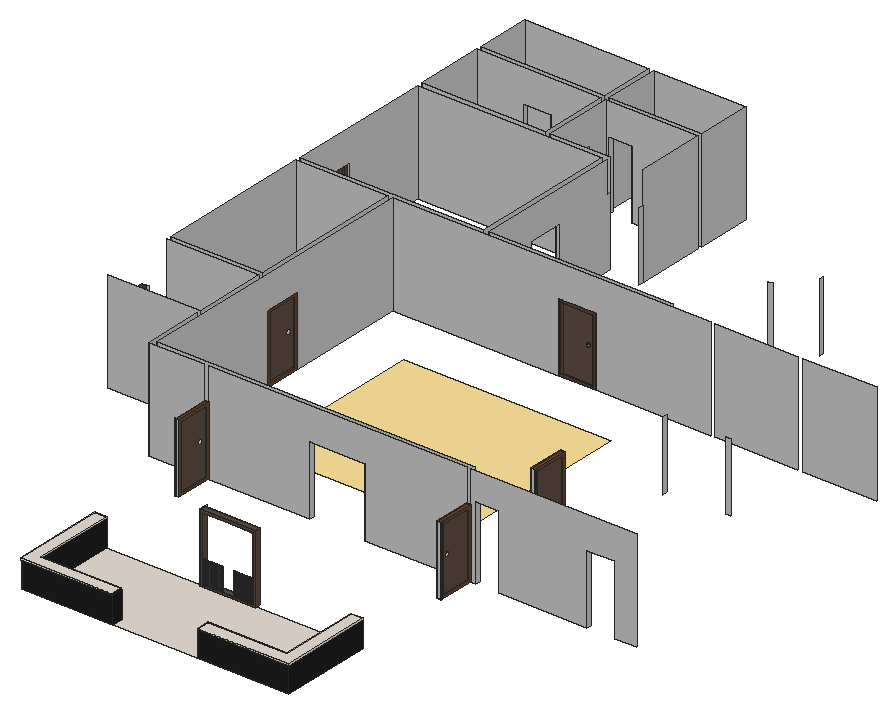
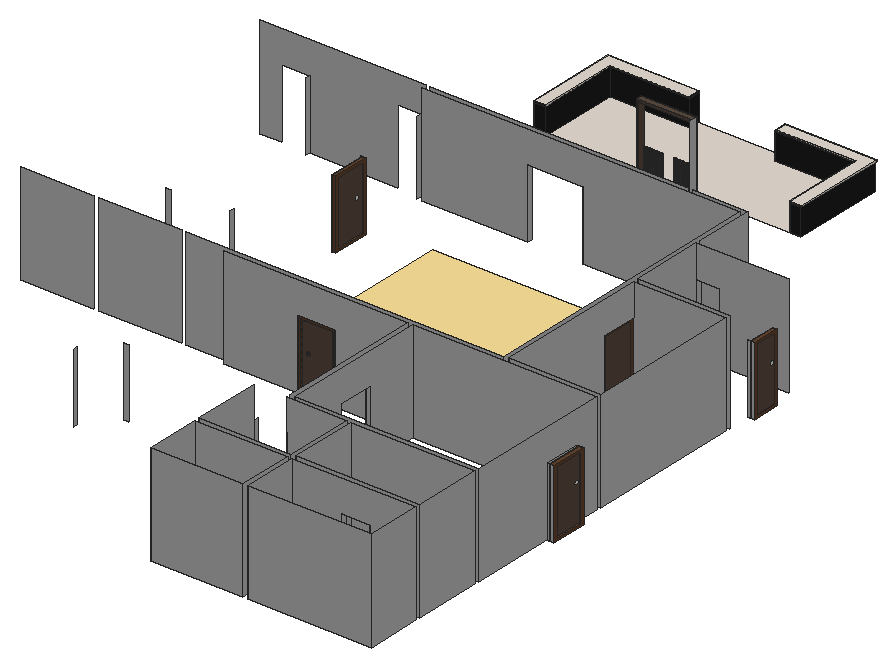
# SketchUp Ruby script. Lengths in inches.
U = 1.inch
M = Sketchup.active_model
def pt(a) = Geom::Point3d.new(a.map { |v| v * U })
def face(e, loops, mat)
  f = e.add_face(loops[0].map { |a| pt(a) })
  loops[1..].each { |l| e.add_face(l.map { |a| pt(a) }).erase! }
  f.material = f.back_material = mat if mat
  f
end
# faces: each face lists its corners as indices into pts; further lists are holes
def faces(e, pts, list, mat = nil) = list.each { |f| face(e, (f[0].is_a?(Array) ? f : [f]).map { |l| l.map { |i| pts[i] } }, mat) }
# xy, xz, yz: faces in a plane at the given z, y or x. An outline is a flat list of corners, or four numbers for a rectangle; further outlines are holes
def ring(l) = l.size == 4 ? [[l[0], l[1]], [l[2], l[1]], [l[2], l[3]], [l[0], l[3]]] : l.each_slice(2).to_a
def flat(e, list, mat, &to3) = list.each { |f| face(e, (f[0].is_a?(Array) ? f : [f]).map { |l| ring(l).map { |u, v| to3.(u, v) } }, mat) }
def xy(e, z, list, mat = nil) = flat(e, list, mat) { |x, y| [x, y, z] }
def xz(e, y, list, mat = nil) = flat(e, list, mat) { |x, z| [x, y, z] }
def yz(e, x, list, mat = nil) = flat(e, list, mat) { |y, z| [x, y, z] }
def lines(e, pts, list) = list.each { |a, b| e.add_line(pt(pts[a]), pt(pts[b])) }
# prism: a flat outline (further loops are holes) pulled along v
def prism(e, loops, v, mat = nil)
  f = face(e, loops, mat); d = Geom::Vector3d.new(v.map { |x| x * U })
  f.pushpull(f.normal.samedirection?(d) ? d.length : -d.length)
end
def box(e, o, s, mat = nil) = prism(e, [[o, [o[0] + s[0], o[1], o[2]], [o[0] + s[0], o[1] + s[1], o[2]], [o[0], o[1] + s[1], o[2]]]], [0, 0, s[2]], mat)
def at(x, y, z, deg = 0) = Geom::Transformation.translation(pt([x, y, z])) * Geom::Transformation.rotation(ORIGIN, Z_AXIS, deg.degrees)
def axes(o, x, y, z) = Geom::Transformation.new([*x, 0, *y, 0, *z, 0, *pt(o).to_a, 1])
def part(name) = M.definitions.add(name)
# library, detail: a bought-in or finely detailed component or shape, given as its bounding box
def library(name, o, s) = part(name).tap { |d| box(d.entities, o, s) }
def detail(e, o, s) = box(e.add_group.entities, o, s)
def put(e, d, t, mat = nil) = e.add_instance(d, t).tap { |i| i.material = mat if mat }
def group(e, t, mat = nil) = e.add_group.tap { |g| g.transformation = t; g.material = mat if mat }.entities
root = M.entities
M.materials.add("Brick_20_1K").color = [126, 109, 93]
M.materials.add("D02_Buttercup_Glow").color = [255, 229, 155]
M.materials.add("M02_Ash_Whisper").color = [196, 196, 196]
M.materials.add("M08_Obsidian_Black").color = [30, 30, 30]
M.materials.add("Marble_01_1K").color = [230, 221, 211]
M.materials.add("Metal_06_1K").color = [238, 236, 231]
M.materials.add("Wood_Floor_12_1K").color = [92, 75, 65]
M.materials.add("Wood_Planks_01_1K").color = [69, 67, 63]
M.materials.add("Wood_Veneer_15_1K").color = [103, 69, 45]
c1 = part("Group\#23")
box(c1.entities,[0,0,0],[0.6875,0.6875,26],"Wood_Planks_01_1K")
c2 = part("Group\#24")
box(c2.entities,[0,0,0],[0.6875,0.75,29.38],"Wood_Planks_01_1K")
c3 = part("Group\#19")
xy(c3.entities,0,[[0,-5,48,0]],"Wood_Veneer_15_1K")
xy(c3.entities,3,[[3,-5,45,-2],[3,-2,45,0]],"Wood_Veneer_15_1K")
xy(c3.entities,87,[[3,-5,45,-2],[3,-2,45,0]],"Wood_Veneer_15_1K")
xy(c3.entities,90,[[0,-5,48,0]],"Wood_Veneer_15_1K")
xz(c3.entities,-5,[[[0,0,48,90],[3,3,45,87]]],"Wood_Veneer_15_1K")
xz(c3.entities,-2,[[3,3,45,87]],"Wood_Floor_12_1K")
xz(c3.entities,0,[[[0,0,48,90],[3,3,45,87]]],"Wood_Veneer_15_1K")
yz(c3.entities,0,[[-5,0,0,90]],"Wood_Veneer_15_1K")
yz(c3.entities,3,[[-5,3,-2,87],[-2,3,0,87]],"Wood_Veneer_15_1K")
yz(c3.entities,45,[[-5,3,-2,87],[-2,3,0,87]],"Wood_Veneer_15_1K")
yz(c3.entities,48,[[-5,0,0,90]],"Wood_Veneer_15_1K")
g1 = group(c3.entities,at(34.34,-2,45.51))
prism(g1,[[[4.08,0,1.09],[3.73,0,0.64],[3.28,0,0.29],[2.75,0,0.07],[2.1875,0,0],[1.62,0,0.07],[1.09,0,0.29],[0.64,0,0.64],[0.29,0,1.09],[0.07,0,1.62],[0,0,2.1875],[0.07,0,2.75],[0.29,0,3.28],[0.64,0,3.73],[1.09,0,4.08],[1.62,0,4.3],[2.1875,0,4.375],[2.75,0,4.3],[3.28,0,4.08],[3.73,0,3.73],[4.08,0,3.28],[4.3,0,2.75],[4.375,0,2.1875],[4.3,0,1.62]]],[0,-0.5625,0],"Metal_06_1K")
c4 = part("Group\#27")
xy(c4.entities,0,[[-6,0,0,36]],"Wood_Veneer_15_1K")
xy(c4.entities,3,[[-3.75,3,0,33]],"Wood_Floor_12_1K")
xy(c4.entities,3,[[-6,3,-3.75,33]],"Wood_Veneer_15_1K")
xy(c4.entities,87,[[-3.75,3,0,33]],"Wood_Floor_12_1K")
xy(c4.entities,87,[[-6,3,-3.75,33]],"Wood_Veneer_15_1K")
xy(c4.entities,90,[[-6,0,0,36]],"Wood_Veneer_15_1K")
xz(c4.entities,0,[[-6,0,0,90]],"Wood_Veneer_15_1K")
xz(c4.entities,3,[[-3.75,3,0,87]],"Wood_Floor_12_1K")
xz(c4.entities,3,[[-6,3,-3.75,87]],"Wood_Veneer_15_1K")
xz(c4.entities,33,[[-3.75,3,0,87]],"Wood_Floor_12_1K")
xz(c4.entities,33,[[-6,3,-3.75,87]],"Wood_Veneer_15_1K")
xz(c4.entities,36,[[-6,0,0,90]],"Wood_Veneer_15_1K")
yz(c4.entities,-6,[[[0,0,36,90],[3,3,33,87]]],"Wood_Veneer_15_1K")
yz(c4.entities,-3.75,[[3,3,33,87]],"Wood_Floor_12_1K")
yz(c4.entities,0,[[[0,0,36,90],[3,3,33,87]]],"Wood_Veneer_15_1K")
g2 = group(c4.entities,at(-3.75,8.7,51.05))
prism(g2,[[[0,-0.26,0.97],[0,-0.07,1.4375],[0,0,1.9375],[0,-0.07,2.4375],[0,-0.26,2.91],[0,-0.57,3.31],[0,-0.97,3.62],[0,-1.4375,3.81],[0,-1.9375,3.875],[0,-2.4375,3.81],[0,-2.91,3.62],[0,-3.31,3.31],[0,-3.62,2.91],[0,-3.81,2.4375],[0,-3.875,1.9375],[0,-3.81,1.4375],[0,-3.62,0.97],[0,-3.31,0.57],[0,-2.91,0.26],[0,-2.4375,0.07],[0,-1.9375,0],[0,-1.4375,0.07],[0,-0.97,0.26],[0,-0.57,0.57]]],[-0.5,0,0],"Metal_06_1K")
xy(root,36,[[2641.48,1061.69,2911.48,1301.69]],"D02_Buttercup_Glow")
xy(root,36,[[2635.48,686.69,2983.48,806.69]],"Marble_01_1K")
xz(root,935.69,[[2635.48,36,2641.48,126],[2977.48,36,2983.48,126]],"M02_Ash_Whisper")
xz(root,983.69,[[2563.48,36,2773.48,36,2773.48,126,2845.48,126,2845.48,36,2989.48,36,2989.48,132,3019.48,132,3019.48,36,3134.81,36,3134.81,126,3170.57,126,3170.57,36,3199.48,36,3199.48,168,2983.48,168,2983.48,126,2977.48,126,2977.48,168,2641.48,168,2641.48,126,2635.48,126,2635.48,168,2563.48,168]],"M02_Ash_Whisper")
xz(root,989.69,[[2569.48,36,2569.48,168,2983.48,168,2983.48,36,2845.48,36,2845.48,126,2773.48,126,2773.48,36]],"M02_Ash_Whisper")
xz(root,1067.69,[[2443.48,36,2443.48,168,2563.48,168,2563.48,36,2562.36,36,2562.36,126,2532.36,126,2532.36,36]],"M02_Ash_Whisper")
xz(root,1081.39,[[2983.48,36,2989.48,126]],"M02_Ash_Whisper")
xz(root,1133.3,[[2434.48,36,2443.48,126]],"M02_Ash_Whisper")
xz(root,1163.69,[[2443.48,36,2563.48,168]],"M02_Ash_Whisper")
xz(root,1169.69,[[2443.48,36,2563.48,168],[2563.48,36,2569.48,126]],"M02_Ash_Whisper")
xz(root,1217.69,[[2563.48,36,2569.48,126]],"M02_Ash_Whisper")
xz(root,1256.05,[[3097.48,36,3103.48,126]],"M02_Ash_Whisper")
xz(root,1373.69,[[2443.48,36,2563.48,168],[2569.48,36,2785.48,36,2785.48,126,2833.48,126,2833.48,36,2983.48,36,2983.48,168,2569.48,168],[2989.48,36,3097.48,168],[3103.48,36,3199.48,168]],"M02_Ash_Whisper")
xz(root,1379.69,[[2443.48,36,2683.48,168],[2689.48,36,2689.48,168,2929.48,168,2929.48,36,2833.48,36,2833.48,126,2785.48,126,2785.48,36]],"M02_Ash_Whisper")
xz(root,1412.46,[[2434.48,36,2443.48,126]],"M02_Ash_Whisper")
xz(root,1448.15,[[2683.48,36,2689.48,126]],"M02_Ash_Whisper")
xz(root,1460.46,[[2434.48,36,2443.48,126]],"M02_Ash_Whisper")
xz(root,1496.15,[[2683.48,36,2689.48,126]],"M02_Ash_Whisper")
xz(root,1534.97,[[2929.48,36,2935.48,126]],"M02_Ash_Whisper")
xz(root,1571.69,[[2443.48,36,2683.48,168]],"M02_Ash_Whisper")
xz(root,1577.69,[[2443.48,36,2605.48,168],[2611.48,36,2689.48,168]],"M02_Ash_Whisper")
xz(root,1615.16,[[2605.48,36,2611.48,126]],"M02_Ash_Whisper")
xz(root,1641.35,[[2605.48,36,2611.48,126]],"M02_Ash_Whisper")
xz(root,1667.69,[[2443.48,36,2504.32,36,2504.32,126,2540.32,126,2540.32,36,2605.48,36,2605.48,168,2443.48,168],[2611.48,36,2615.5625,36,2615.5625,126,2645.5625,126,2645.5625,36,2731.48,36,2731.48,168,2611.48,168]],"M02_Ash_Whisper")
xz(root,1673.69,[[2443.48,36,2443.48,168,2605.48,168,2605.48,36,2540.32,36,2540.32,126,2504.32,126,2504.32,36],[2611.48,36,2611.48,168,2731.48,168,2731.48,36,2645.5625,36,2645.5625,126,2615.5625,126,2615.5625,36]],"M02_Ash_Whisper")
xz(root,1745.69,[[2443.48,36,2605.48,168],[2611.48,36,2731.48,168]],"M02_Ash_Whisper")
yz(root,2443.48,[[1169.69,36,1373.69,168],[1379.69,36,1412.46,36,1412.46,126,1460.46,126,1460.46,36,1571.69,36,1571.69,168,1379.69,168],[1577.69,36,1667.69,168],[1673.69,36,1745.69,168]],"M02_Ash_Whisper")
yz(root,2504.32,[[1667.69,36,1673.69,126]],"M02_Ash_Whisper")
yz(root,2540.32,[[1667.69,36,1673.69,126]],"M02_Ash_Whisper")
yz(root,2562.36,[[1061.69,36,1067.69,126]],"M02_Ash_Whisper")
yz(root,2563.48,[[983.69,36,1061.69,168],[1067.69,36,1163.69,168],[1217.69,36,1217.69,126,1169.69,126,1169.69,168,1373.69,168,1373.69,36]],"M02_Ash_Whisper")
yz(root,2569.48,[[989.69,36,1169.69,36,1169.69,126,1217.69,126,1217.69,36,1373.69,36,1373.69,168,989.69,168]],"M02_Ash_Whisper")
yz(root,2605.48,[[1577.69,36,1577.69,168,1667.69,168,1667.69,36,1641.35,36,1641.35,126,1615.16,126,1615.16,36],[1673.69,36,1745.69,168]],"M02_Ash_Whisper")
yz(root,2611.48,[[1577.69,36,1615.16,36,1615.16,126,1641.35,126,1641.35,36,1667.69,36,1667.69,168,1577.69,168],[1673.69,36,1745.69,168]],"M02_Ash_Whisper")
yz(root,2615.5625,[[1667.69,36,1673.69,126]],"M02_Ash_Whisper")
yz(root,2645.5625,[[1667.69,36,1673.69,126]],"M02_Ash_Whisper")
yz(root,2683.48,[[1379.69,36,1379.69,168,1571.69,168,1571.69,36,1496.15,36,1496.15,126,1448.15,126,1448.15,36]],"M02_Ash_Whisper")
yz(root,2689.48,[[1379.69,36,1448.15,36,1448.15,126,1496.15,126,1496.15,36,1577.69,36,1577.69,126,1571.69,126,1571.69,168,1379.69,168]],"M02_Ash_Whisper")
yz(root,2731.48,[[1571.69,36,1577.69,126],[1577.69,36,1667.69,168],[1673.69,36,1745.69,168]],"M02_Ash_Whisper")
yz(root,2773.48,[[806.69,36,815.69,126],[983.69,36,989.69,126]],"M02_Ash_Whisper")
yz(root,2785.48,[[1373.69,36,1379.69,126]],"M02_Ash_Whisper")
yz(root,2833.48,[[1373.69,36,1379.69,126]],"M02_Ash_Whisper")
yz(root,2845.48,[[983.69,36,989.69,126]],"M02_Ash_Whisper")
yz(root,2967.08,[[1571.69,36,1577.69,126]],"M02_Ash_Whisper")
yz(root,2989.48,[[983.69,36,989.69,132]],"M02_Ash_Whisper")
yz(root,3021.96,[[1247.69,36,1253.69,126]],"M02_Ash_Whisper")
yz(root,3134.81,[[983.69,36,989.69,126]],"M02_Ash_Whisper")
g3 = group(root,at(2635.48,686.69,36),"Brick_20_1K")
xy(g3,0,[[0,0,0,120,14.5,120,14.5,13.81,118.8125,13.81,118.8125,0]],"M08_Obsidian_Black")
xy(g3,34.69,[[0,0,0,120,14.5,120,14.5,13.81,117.8125,13.81,117.8125,0],[117.8125,0,118.8125,13.81]],"M08_Obsidian_Black")
xy(g3,34.69,[[-1,-1,117.8125,0],[-1,0,0,120]],"Marble_01_1K")
xy(g3,36.69,[[-1,-1,117.8125,-1,117.8125,13.81,14.5,13.81,14.5,120,-1,120]],"Marble_01_1K")
xz(g3,-1,[[-1,34.69,117.8125,36.69]],"Marble_01_1K")
xz(g3,0,[[0,0,118.8125,34.69]],"M08_Obsidian_Black")
xz(g3,13.81,[[14.5,0,118.8125,34.69]],"M08_Obsidian_Black")
xz(g3,13.81,[[14.5,34.69,117.8125,36.69]],"Marble_01_1K")
xz(g3,120,[[0,0,14.5,34.69],[-1,34.69,14.5,36.69]],"M08_Obsidian_Black")
yz(g3,-1,[[-1,34.69,120,36.69]],"Marble_01_1K")
yz(g3,0,[[0,0,120,34.69]],"M08_Obsidian_Black")
yz(g3,14.5,[[13.81,0,120,34.69]],"M08_Obsidian_Black")
yz(g3,14.5,[[13.81,34.69,120,36.69]],"Marble_01_1K")
yz(g3,117.8125,[[-1,34.69,13.81,36.69]],"M08_Obsidian_Black")
yz(g3,118.8125,[[0,0,13.81,34.69]],"M08_Obsidian_Black")
g4 = group(root,at(2974.48,686.69,36),"Brick_20_1K")
xy(g4,0,[[-109.0625,0,-109.0625,14.5,-5.5,14.5,-5.5,120,9,120,9,0]],"M08_Obsidian_Black")
xy(g4,34,[[-109.0625,0,-108.0625,14.5],[-108.0625,0,-108.0625,14.5,-5.5,14.5,-5.5,120,9,120,9,0]],"M08_Obsidian_Black")
xy(g4,34,[[-108.0625,-1.69,10,0],[9,0,10,120]],"Marble_01_1K")
xy(g4,36,[[-108.0625,-1.69,10,-1.69,10,120,-5.5,120,-5.5,14.5,-108.0625,14.5]],"Marble_01_1K")
xz(g4,-1.69,[[-108.0625,34,10,36]],"Marble_01_1K")
xz(g4,0,[[-109.0625,0,9,34]],"M08_Obsidian_Black")
xz(g4,14.5,[[-109.0625,0,-5.5,34]],"M08_Obsidian_Black")
xz(g4,14.5,[[-108.0625,34,-5.5,36]],"Marble_01_1K")
xz(g4,120,[[-5.5,0,9,34],[-5.5,34,10,36]],"M08_Obsidian_Black")
yz(g4,-109.0625,[[0,0,14.5,34]],"M08_Obsidian_Black")
yz(g4,-108.0625,[[-1.69,34,14.5,36]],"M08_Obsidian_Black")
yz(g4,-5.5,[[14.5,0,120,34]],"M08_Obsidian_Black")
yz(g4,-5.5,[[14.5,34,120,36]],"Marble_01_1K")
yz(g4,9,[[0,0,120,34]],"M08_Obsidian_Black")
yz(g4,10,[[-1.69,34,120,36]],"Marble_01_1K")
g5 = group(root,at(2773.48,812.69,36),"Brick_20_1K")
prism(g5,[[[72,0,90],[72,0,0],[0,0,0],[0,0,90]],[[3,0,3],[69,0,3],[69,0,87],[35,0,87],[3,0,87]]],[0,-7.9375,0],"Wood_Floor_12_1K")
put(g5,c1,axes([3,-7.52,31.7],[0,1,0],[0,0,1],[1,0,0]))
put(g5,c1,axes([3,-7.52,28.98],[0,1,0],[0,0,1],[1,0,0]))
put(g5,c1,axes([3,-7.52,26.27],[0,1,0],[0,0,1],[1,0,0]))
put(g5,c1,axes([3,-7.52,23.56],[0,1,0],[0,0,1],[1,0,0]))
put(g5,c1,axes([3,-7.52,20.85],[0,1,0],[0,0,1],[1,0,0]))
put(g5,c1,axes([3,-7.52,18.13],[0,1,0],[0,0,1],[1,0,0]))
put(g5,c1,axes([3,-7.52,15.42],[0,1,0],[0,0,1],[1,0,0]))
put(g5,c1,axes([3,-7.52,12.71],[0,1,0],[0,0,1],[1,0,0]))
put(g5,c1,axes([3,-7.52,10],[0,1,0],[0,0,1],[1,0,0]))
put(g5,c1,axes([3,-7.52,7.28],[0,1,0],[0,0,1],[1,0,0]))
put(g5,c1,axes([3,-7.52,4.57],[0,1,0],[0,0,1],[1,0,0]))
put(g5,c2,at(4.03,-7.58,3))
put(g5,c2,at(6.37,-7.58,3))
put(g5,c2,at(8.71,-7.58,3))
put(g5,c2,at(11.04,-7.58,3))
put(g5,c2,at(13.38,-7.58,3))
put(g5,c2,at(15.72,-7.58,3))
put(g5,c2,at(18.06,-7.58,3))
put(g5,c2,at(20.39,-7.58,3))
put(g5,c2,at(22.73,-7.58,3))
put(g5,c2,at(25.07,-7.58,3))
put(g5,c2,at(27.41,-7.58,3))
put(g5,c1,axes([43,-7.52,10],[0,1,0],[0,0,1],[1,0,0]))
put(g5,c1,axes([43,-7.52,4.57],[0,1,0],[0,0,1],[1,0,0]))
put(g5,c2,at(44.03,-7.58,3))
put(g5,c1,axes([43,-7.52,15.42],[0,1,0],[0,0,1],[1,0,0]))
put(g5,c1,axes([43,-7.52,12.71],[0,1,0],[0,0,1],[1,0,0]))
put(g5,c1,axes([43,-7.52,26.27],[0,1,0],[0,0,1],[1,0,0]))
put(g5,c1,axes([43,-7.52,20.85],[0,1,0],[0,0,1],[1,0,0]))
put(g5,c1,axes([43,-7.52,23.56],[0,1,0],[0,0,1],[1,0,0]))
put(g5,c1,axes([43,-7.52,28.98],[0,1,0],[0,0,1],[1,0,0]))
put(g5,c1,axes([43,-7.52,7.28],[0,1,0],[0,0,1],[1,0,0]))
put(g5,c1,axes([43,-7.52,18.13],[0,1,0],[0,0,1],[1,0,0]))
put(g5,c1,axes([43,-7.52,31.7],[0,1,0],[0,0,1],[1,0,0]))
put(g5,c2,at(67.41,-7.58,3))
put(g5,c2,at(53.38,-7.58,3))
put(g5,c2,at(58.06,-7.58,3))
put(g5,c2,at(60.39,-7.58,3))
put(g5,c2,at(48.71,-7.58,3))
put(g5,c2,at(46.37,-7.58,3))
put(g5,c2,at(62.73,-7.58,3))
put(g5,c2,at(65.07,-7.58,3))
put(g5,c2,at(55.72,-7.58,3))
put(g5,c2,at(51.04,-7.58,3))
put(root,c3,at(2785.48,1378.69,36))
put(root,c3,at(2564.48,1169.69,36,90))
put(root,c3,at(2988.48,1129.39,36,-90))
put(root,c3,at(2636.48,935.69,36,90))
put(root,c3,at(2982.48,983.69,36,-90))
put(root,c4,at(2440.48,1097.3,36))
put(root,c4,axes([2440.48,1412.72,36],[1,0,0],[0,1.326,0],[0,0,1]))
